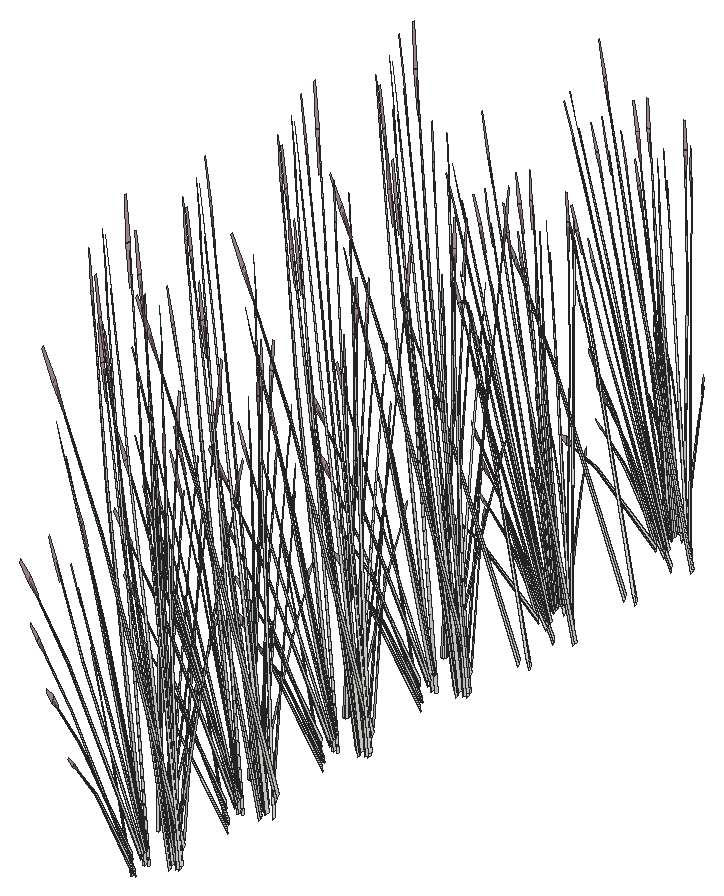
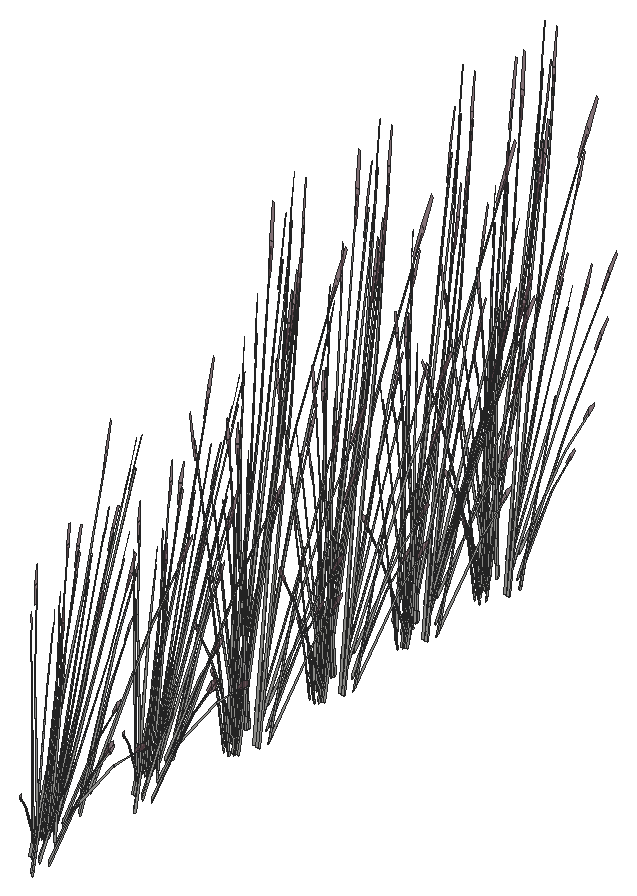
# SketchUp Ruby script. Lengths in inches.
U = 1.inch
M = Sketchup.active_model
def pt(a) = Geom::Point3d.new(a.map { |v| v * U })
def face(e, loops, mat)
  f = e.add_face(loops[0].map { |a| pt(a) })
  loops[1..].each { |l| e.add_face(l.map { |a| pt(a) }).erase! }
  f.material = f.back_material = mat if mat
  f
end
# faces: each face lists its corners as indices into pts; further lists are holes
def faces(e, pts, list, mat = nil) = list.each { |f| face(e, (f[0].is_a?(Array) ? f : [f]).map { |l| l.map { |i| pts[i] } }, mat) }
# xy, xz, yz: faces in a plane at the given z, y or x. An outline is a flat list of corners, or four numbers for a rectangle; further outlines are holes
def ring(l) = l.size == 4 ? [[l[0], l[1]], [l[2], l[1]], [l[2], l[3]], [l[0], l[3]]] : l.each_slice(2).to_a
def flat(e, list, mat, &to3) = list.each { |f| face(e, (f[0].is_a?(Array) ? f : [f]).map { |l| ring(l).map { |u, v| to3.(u, v) } }, mat) }
def xy(e, z, list, mat = nil) = flat(e, list, mat) { |x, y| [x, y, z] }
def xz(e, y, list, mat = nil) = flat(e, list, mat) { |x, z| [x, y, z] }
def yz(e, x, list, mat = nil) = flat(e, list, mat) { |y, z| [x, y, z] }
def lines(e, pts, list) = list.each { |a, b| e.add_line(pt(pts[a]), pt(pts[b])) }
# prism: a flat outline (further loops are holes) pulled along v
def prism(e, loops, v, mat = nil)
  f = face(e, loops, mat); d = Geom::Vector3d.new(v.map { |x| x * U })
  f.pushpull(f.normal.samedirection?(d) ? d.length : -d.length)
end
def box(e, o, s, mat = nil) = prism(e, [[o, [o[0] + s[0], o[1], o[2]], [o[0] + s[0], o[1] + s[1], o[2]], [o[0], o[1] + s[1], o[2]]]], [0, 0, s[2]], mat)
def at(x, y, z, deg = 0) = Geom::Transformation.translation(pt([x, y, z])) * Geom::Transformation.rotation(ORIGIN, Z_AXIS, deg.degrees)
def axes(o, x, y, z) = Geom::Transformation.new([*x, 0, *y, 0, *z, 0, *pt(o).to_a, 1])
def part(name) = M.definitions.add(name)
# library, detail: a bought-in or finely detailed component or shape, given as its bounding box
def library(name, o, s) = part(name).tap { |d| box(d.entities, o, s) }
def detail(e, o, s) = box(e.add_group.entities, o, s)
def put(e, d, t, mat = nil) = e.add_instance(d, t).tap { |i| i.material = mat if mat }
def group(e, t, mat = nil) = e.add_group.tap { |g| g.transformation = t; g.material = mat if mat }.entities
root = M.entities
M.materials.add("LightPink_Translucent").color = [144, 107, 117]
M.materials["LightPink_Translucent"].alpha = 0.75
c1 = part("blade")
p = [[2.15,0.21,22],[0,0.17,0],[0.09,0.45,0],[2.18,0.31,22],[2.29,0.31,22],[0.38,0.45,0],
  [2.48,0.24,33],[2.49,0.24,33],[2.48,0.22,33]]
faces(c1.entities,p,[[0,1,2,3],[4,5,2,3],[6,3,4,7],[8,0,3,6]])
c2 = part("seeds")
p = [[0.3,-0.1,1.38],[-0.01,-0.03,1.59],[-0.01,-0.03,0.03],[0.14,-0.07,-0.07],[0.29,-0.03,3],[0.15,0.01,3.11]]
faces(c2.entities,p,[[0,1,2,3],[1,0,4,5]],"LightPink_Translucent")
c3 = part("blade with seeds")
put(c3.entities,c1,at(0,0,0))
put(c3.entities,c2,axes([2.4,0.25,30.99],[1.5799,-0.05474,1.17369],[-0.12525,1.92788,0.29478],[-0.07173,-0.02425,1.56792]))
put(root,c3,axes([402.11,21.07,-7.6],[0.02575,-0.41332,0.05988],[0.38885,0.01133,0.47138],[-0.14895,-0.04325,0.71878]))
put(root,c3,axes([402.13,36.38,-10.12],[-0.47863,-0.27177,-0.46235],[0.28609,-0.48733,0],[-0.10901,-0.0619,1.46668]))
put(root,c3,axes([401.1875,24.6,-7.61],[-0.01271,0.10756,1.62908],[0.36076,0.37419,-0.25764],[-0.09444,0.17695,0.13065]))
put(root,c3,axes([402.15,48.24,-10.12],[-0.47863,-0.27177,-0.46235],[0.28609,-0.48733,0],[-0.10901,-0.0619,1.46668]))
put(root,c3,axes([401.92,32.34,-10.61],[-0.04954,0.0716,1.6421],[-0.50062,0.15438,-0.25086],[-0.12094,-0.14044,0.2797]))
put(root,c3,axes([401.36,35.34,-7.3125],[0.47307,0.29971,-0.11324],[-0.27254,0.43404,-0.62851],[-0.13365,0.15087,0.95501]))
put(root,c3,axes([401.94,44.19,-10.61],[-0.04954,0.0716,1.6421],[-0.50062,0.15438,-0.25086],[-0.12094,-0.14044,0.2797]))
put(root,c3,axes([401.38,47.2,-7.3125],[0.47307,0.29971,-0.11324],[-0.27254,0.43404,-0.62851],[-0.13365,0.15087,0.95501]))
put(root,c3,axes([403.21,23.36,-10.08],[-0.53199,-0.08911,-0.58063],[0.11226,-0.54969,-0.15239],[-0.15876,-0.06661,1.28164]))
put(root,c3,axes([403.3,20.36,-6.94],[-0.34131,0.52108,-0.12682],[-0.49429,-0.3002,-0.70393],[-0.17182,-0.14722,1.06961]))
put(root,c3,axes([400.33,14.06,-6.74],[0.45129,0.14509,-0.06041],[-0.13882,0.44656,-0.27392],[-0.07381,0.0678,0.90349]))
put(root,c3,axes([402.42,36.71,-9.79],[-0.31974,0.54466,0],[-0.53494,-0.30375,-0.48057],[-0.12184,-0.06918,1.52448]))
put(root,c3,axes([402.37,21.38,-7.3],[0.29098,0.34031,0.32977],[-0.33226,0.32215,-0.42575],[-0.16881,-0.04902,0.81462]))
put(root,c3,axes([401.95,73.36,-7.62],[0.06527,0.01458,1.65179],[0.20191,0.48025,-0.15608],[-0.1336,0.12605,0.29231]))
put(root,c3,axes([402.45,48.57,-9.79],[-0.31974,0.54466,0],[-0.53494,-0.30375,-0.48057],[-0.12184,-0.06918,1.52448]))
put(root,c3,axes([401.96,59.11,-7.62],[0.06527,0.01458,1.65179],[0.20191,0.48025,-0.15608],[-0.1336,0.12605,0.29231]))
put(root,c3,axes([403.4375,72.77,-7.64],[-0.13855,0.49442,-0.47583],[-0.47502,-0.16947,-0.36857],[-0.19125,0.04534,0.91046]))
put(root,c3,axes([403.44,58.52,-7.64],[-0.13855,0.49442,-0.47583],[-0.47502,-0.16947,-0.36857],[-0.19125,0.04534,0.91046]))
put(root,c3,axes([401.34,12.8,-7.3],[0.44516,-0.07768,0.32977],[0.11755,0.44407,-0.42575],[-0.12757,0.11927,0.81462]))
put(root,c3,axes([403.15,20.78,-7.36],[-0.43608,-0.26272,-0.66157],[0.30991,-0.46038,0.07984],[-0.158,-0.15687,0.93586]))
put(root,c3,axes([402.95,20.79,-7.64],[-0.50465,0.12921,-0.47583],[-0.08828,-0.48932,-0.36857],[-0.13555,-0.14022,0.91046]))
put(root,c3,axes([401.6,14.92,-9.59],[0.16138,-0.08575,1.33163],[0.39845,0.25854,-0.28638],[-0.1186,0.22371,0.56934]))
put(root,c3,axes([403.8,71.7,-7.64],[-0.37135,0.36005,-0.47583],[-0.32522,-0.38035,-0.36857],[-0.18868,-0.05478,0.91046]))
put(root,c3,axes([403.8,57.46,-7.64],[-0.37135,0.36005,-0.47583],[-0.32522,-0.38035,-0.36857],[-0.18868,-0.05478,0.91046]))
put(root,c3,axes([403.2,72.74,-10.61],[0.01297,0.08566,1.6421],[-0.26146,0.44735,-0.25086],[-0.18572,-0.02255,0.2797]))
put(root,c3,axes([403.21,58.49,-10.61],[0.01297,0.08566,1.6421],[-0.26146,0.44735,-0.25086],[-0.18572,-0.02255,0.2797]))
put(root,c3,axes([401.37,10.03,-10.02],[-0.14753,0.44383,-0.03625],[-0.45406,-0.13653,-0.16435],[-0.06894,-0.07259,0.54209]))
put(root,c3,axes([400.58,36.65,-6.74],[0.45129,0.14509,-0.06041],[-0.13882,0.44656,-0.27392],[-0.07381,0.0678,0.90349]))
put(root,c3,axes([400.6,48.5,-6.74],[0.45129,0.14509,-0.06041],[-0.13882,0.44656,-0.27392],[-0.07381,0.0678,0.90349]))
put(root,c3,axes([402.51,24.4,-10.12],[-0.47863,-0.27177,-0.46235],[0.28609,-0.48733,0],[-0.10901,-0.0619,1.46668]))
put(root,c3,axes([402.55,8.52,-7.62],[-0.00954,0.06515,1.65179],[-0.47055,0.23645,-0.15608],[-0.13847,-0.12087,0.29231]))
put(root,c3,axes([402.3,20.35,-10.61],[-0.04954,0.0716,1.6421],[-0.50062,0.15438,-0.25086],[-0.12094,-0.14044,0.2797]))
put(root,c3,axes([401.73,23.36,-7.3125],[0.47307,0.29971,-0.11324],[-0.27254,0.43404,-0.62851],[-0.13365,0.15087,0.95501]))
put(root,c3,axes([403.27,70.69,-7.62],[0.03791,0.05424,1.65179],[-0.18278,0.48761,-0.15608],[-0.18511,0.00353,0.29231]))
put(root,c3,axes([401.59,35.38,-7.3],[0.44516,-0.07768,0.32977],[0.11755,0.44407,-0.42575],[-0.12757,0.11927,0.81462]))
put(root,c3,axes([403.28,56.45,-7.62],[0.03791,0.05424,1.65179],[-0.18278,0.48761,-0.15608],[-0.18511,0.00353,0.29231]))
put(root,c3,axes([401.61,47.24,-7.3],[0.44516,-0.07768,0.32977],[0.11755,0.44407,-0.42575],[-0.12757,0.11927,0.81462]))
put(root,c3,axes([402.05,9.47,-9.59],[-0.03097,0.17781,1.33163],[-0.45273,0.14885,-0.28638],[-0.10583,-0.22982,0.56934]))
put(root,c3,axes([401.84,37.5,-9.59],[0.16138,-0.08575,1.33163],[0.39845,0.25854,-0.28638],[-0.1186,0.22371,0.56934]))
put(root,c3,axes([402.8,24.72,-9.79],[-0.31974,0.54466,0],[-0.53494,-0.30375,-0.48057],[-0.12184,-0.06918,1.52448]))
put(root,c3,axes([401.86,49.36,-9.59],[0.16138,-0.08575,1.33163],[0.39845,0.25854,-0.28638],[-0.1186,0.22371,0.56934]))
put(root,c3,axes([402.5,74.88,-9.42],[0.21313,-0.24635,1.06958],[0.0841,0.38999,0.78586],[-0.15402,0.06983,0.23558]))
put(root,c3,axes([402.19,9.93,-8.39],[0.1169,0.17452,1.59586],[-0.54019,0.14692,0.12904],[-0.12209,-0.27397,0.68222]))
put(root,c3,axes([402.51,60.64,-9.42],[0.21313,-0.24635,1.06958],[0.0841,0.38999,0.78586],[-0.15402,0.06983,0.23558]))
put(root,c3,axes([401.61,32.61,-10.02],[-0.14753,0.44383,-0.03625],[-0.45406,-0.13653,-0.16435],[-0.06894,-0.07259,0.54209]))
put(root,c3,axes([403.19,12.84,-9.52],[-0.51635,0.36087,-0.27094],[-0.34336,-0.5099,-0.46562],[-0.1274,-0.05178,1.4872]))
put(root,c3,axes([401.63,44.47,-10.02],[-0.14753,0.44383,-0.03625],[-0.45406,-0.13653,-0.16435],[-0.06894,-0.07259,0.54209]))
put(root,c3,axes([403.7,70.37,-7.61],[-0.11004,-0.00384,1.62908],[-0.35032,0.38367,-0.25764],[-0.18692,-0.07839,0.13065]))
put(root,c3,axes([403.7,56.12,-7.61],[-0.11004,-0.00384,1.62908],[-0.35032,0.38367,-0.25764],[-0.18692,-0.07839,0.13065]))
put(root,c3,axes([401.76,13.98,-7.59],[-0.36417,-0.37086,0.447],[0.38674,-0.31985,0.36857],[-0.06718,0.174,0.92496]))
put(root,c3,axes([402.38,9.84,-7.78],[-0.07899,-0.43781,-0.32977],[0.45153,-0.11561,0.42575],[-0.12128,-0.12546,0.81462]))
put(root,c3,axes([403.25,72.49,-7.59],[0.14449,-0.4956,0.447],[0.47502,0.16947,0.36857],[-0.1868,0.02978,0.92496]))
put(root,c3,axes([402.79,31.11,-7.62],[-0.00954,0.06515,1.65179],[-0.47055,0.23645,-0.15608],[-0.13847,-0.12087,0.29231]))
put(root,c3,axes([403.25,58.24,-7.59],[0.14449,-0.4956,0.447],[0.47502,0.16947,0.36857],[-0.1868,0.02978,0.92496]))
put(root,c3,axes([402.82,42.96,-7.62],[-0.00954,0.06515,1.65179],[-0.47055,0.23645,-0.15608],[-0.13847,-0.12087,0.29231]))
put(root,c3,axes([401.125,12.05,-9.79],[-0.63949,0,0],[0,-0.60749,-0.48057],[0,-0.13836,1.52448]))
put(root,c3,axes([402.02,13.6,-10.11],[-0.12013,-0.47362,-0.28847],[0.47712,-0.13449,0.28847],[-0.09619,-0.05462,1.29413]))
put(root,c3,axes([403.42,72.35,-7.3125],[0.25732,0.49218,-0.11324],[-0.45669,0.24187,-0.62851],[-0.19245,0.06494,0.95501]))
put(root,c3,axes([403.42,58.1,-7.3125],[0.25732,0.49218,-0.11324],[-0.45669,0.24187,-0.62851],[-0.19245,0.06494,0.95501]))
put(root,c3,axes([401.63,13.94,-7.6],[-0.42027,-0.02533,0.05988],[0.01152,-0.38243,0.47138],[-0.04398,0.14649,0.71878]))
put(root,c3,axes([403.99,71.32,-7.3125],[-0.02738,0.55277,-0.11324],[-0.51847,-0.01511,-0.62851],[-0.19968,-0.0384,0.95501]))
put(root,c3,axes([402.29,32.05,-9.59],[-0.03097,0.17781,1.33163],[-0.45273,0.14885,-0.28638],[-0.10583,-0.22982,0.56934]))
put(root,c3,axes([400.95,24.66,-6.74],[0.45129,0.14509,-0.06041],[-0.13882,0.44656,-0.27392],[-0.07381,0.0678,0.90349]))
put(root,c3,axes([404,57.08,-7.3125],[-0.02738,0.55277,-0.11324],[-0.51847,-0.01511,-0.62851],[-0.19968,-0.0384,0.95501]))
put(root,c3,axes([403.66,71.36,-7.78],[-0.29098,-0.34031,-0.32977],[0.33226,-0.32215,0.42575],[-0.16881,-0.04902,0.81462]))
put(root,c3,axes([402.3125,43.91,-9.59],[-0.03097,0.17781,1.33163],[-0.45273,0.14885,-0.28638],[-0.10583,-0.22982,0.56934]))
put(root,c3,axes([403.67,57.12,-7.78],[-0.29098,-0.34031,-0.32977],[0.33226,-0.32215,0.42575],[-0.16881,-0.04902,0.81462]))
put(root,c3,axes([403.21,72.36,-7.6],[-0.18783,-0.37061,0.05988],[0.34252,-0.1814,0.47138],[-0.15099,0.03579,0.71878]))
put(root,c3,axes([403.22,58.11,-7.6],[-0.18783,-0.37061,0.05988],[0.34252,-0.1814,0.47138],[-0.15099,0.03579,0.71878]))
put(root,c3,axes([402.4375,32.51,-8.39],[0.1169,0.17452,1.59586],[-0.54019,0.14692,0.12904],[-0.12209,-0.27397,0.68222]))
put(root,c3,axes([401.76,14.09,-7.78],[-0.34603,0.28618,-0.32977],[-0.32756,-0.32677,0.42575],[-0.04984,0.16603,0.81462]))
put(root,c3,axes([402.46,44.37,-8.39],[0.1169,0.17452,1.59586],[-0.54019,0.14692,0.12904],[-0.12209,-0.27397,0.68222]))
put(root,c3,axes([403.43,35.42,-9.52],[-0.51635,0.36087,-0.27094],[-0.34336,-0.5099,-0.46562],[-0.1274,-0.05178,1.4872]))
put(root,c3,axes([404.07,73.38,-8.39],[0.12773,-0.16701,1.59586],[0.32252,0.4508,0.12904],[-0.22121,0.20529,0.68222]))
put(root,c3,axes([401.96,23.4,-7.3],[0.44516,-0.07768,0.32977],[0.11755,0.44407,-0.42575],[-0.12757,0.11927,0.81462]))
put(root,c3,axes([404.08,59.14,-8.39],[0.12773,-0.16701,1.59586],[0.32252,0.4508,0.12904],[-0.22121,0.20529,0.68222]))
put(root,c3,axes([403.3,73.82,-7.78],[-0.44516,0.07768,-0.32977],[-0.11755,-0.44407,0.42575],[-0.12757,0.11927,0.81462]))
put(root,c3,axes([403.31,59.57,-7.78],[-0.44516,0.07768,-0.32977],[-0.11755,-0.44407,0.42575],[-0.12757,0.11927,0.81462]))
put(root,c3,axes([403.46,47.28,-9.52],[-0.51635,0.36087,-0.27094],[-0.34336,-0.5099,-0.46562],[-0.1274,-0.05178,1.4872]))
put(root,c3,axes([402.01,36.5625,-7.59],[-0.36417,-0.37086,0.447],[0.38674,-0.31985,0.36857],[-0.06718,0.174,0.92496]))
put(root,c3,axes([402.03,48.42,-7.59],[-0.36417,-0.37086,0.447],[0.38674,-0.31985,0.36857],[-0.06718,0.174,0.92496]))
put(root,c3,axes([402.22,25.51,-9.59],[0.16138,-0.08575,1.33163],[0.39845,0.25854,-0.28638],[-0.1186,0.22371,0.56934]))
put(root,c3,axes([402.625,32.42,-7.78],[-0.07899,-0.43781,-0.32977],[0.45153,-0.11561,0.42575],[-0.12128,-0.12546,0.81462]))
put(root,c3,axes([403.06,75.14,-10.61],[0.0686,0.0543,1.6421],[0.11632,0.50315,-0.25086],[-0.15204,0.10729,0.2797]))
put(root,c3,axes([401.99,20.625,-10.02],[-0.14753,0.44383,-0.03625],[-0.45406,-0.13653,-0.16435],[-0.06894,-0.07259,0.54209]))
put(root,c3,axes([402.65,44.28,-7.78],[-0.07899,-0.43781,-0.32977],[0.45153,-0.11561,0.42575],[-0.12128,-0.12546,0.81462]))
put(root,c3,axes([403.07,60.89,-10.61],[0.0686,0.0543,1.6421],[0.11632,0.50315,-0.25086],[-0.15204,0.10729,0.2797]))
put(root,c3,axes([401.37,34.64,-9.79],[-0.63949,0,0],[0,-0.60749,-0.48057],[0,-0.13836,1.52448]))
put(root,c3,axes([403.53,13.23,-10.08],[-0.34446,0.40855,-0.58063],[-0.42791,-0.37046,-0.15239],[-0.13803,0.10191,1.28164]))
put(root,c3,axes([402.27,36.18,-10.11],[-0.12013,-0.47362,-0.28847],[0.47712,-0.13449,0.28847],[-0.09619,-0.05462,1.29413]))
put(root,c3,axes([401.39,46.5,-9.79],[-0.63949,0,0],[0,-0.60749,-0.48057],[0,-0.13836,1.52448]))
put(root,c3,axes([402.96,72.18,-9.42],[0.3265,-0.03889,1.06958],[-0.20711,0.3427,0.78586],[-0.16135,-0.05141,0.23558]))
put(root,c3,axes([402.29,48.04,-10.11],[-0.12013,-0.47362,-0.28847],[0.47712,-0.13449,0.28847],[-0.09619,-0.05462,1.29413]))
put(root,c3,axes([401.875,36.53,-7.6],[-0.42027,-0.02533,0.05988],[0.01152,-0.38243,0.47138],[-0.04398,0.14649,0.71878]))
put(root,c3,axes([402.65,10.19,-7.3],[0.07899,0.43781,0.32977],[-0.45153,0.11561,-0.42575],[-0.12128,-0.12546,0.81462]))
put(root,c3,axes([402.97,57.93,-9.42],[0.3265,-0.03889,1.06958],[-0.20711,0.3427,0.78586],[-0.16135,-0.05141,0.23558]))
put(root,c3,axes([401.9,48.39,-7.6],[-0.42027,-0.02533,0.05988],[0.01152,-0.38243,0.47138],[-0.04398,0.14649,0.71878]))
put(root,c3,axes([400.53,15.11,-7.62],[0.05802,-0.03282,1.65179],[0.47954,0.21828,-0.15608],[-0.01127,0.18175,0.29231]))
put(root,c3,axes([401.62,11.89,-9.83],[-0.47569,0.45698,0.2864],[-0.47598,-0.45217,-0.33981],[-0.01661,-0.12977,1.53541]))
put(root,c3,axes([402.01,36.67,-7.78],[-0.34603,0.28618,-0.32977],[-0.32756,-0.32677,0.42575],[-0.04984,0.16603,0.81462]))
put(root,c3,axes([403.17,19.12,-7.62],[-0.00954,0.06515,1.65179],[-0.47055,0.23645,-0.15608],[-0.13847,-0.12087,0.29231]))
put(root,c3,axes([402.03,48.53,-7.78],[-0.34603,0.28618,-0.32977],[-0.32756,-0.32677,0.42575],[-0.04984,0.16603,0.81462]))
put(root,c3,axes([405.76,50.98,-8.39],[0.21212,-0.01231,1.59586],[-0.14072,0.53355,0.12904],[-0.3023,-0.033,0.68222]))
put(root,c3,axes([405.77,63.82,-8.39],[0.21212,-0.01231,1.59586],[-0.14072,0.53355,0.12904],[-0.3023,-0.033,0.68222]))
put(root,c3,axes([402.66,20.06,-9.59],[-0.03097,0.17781,1.33163],[-0.45273,0.14885,-0.28638],[-0.10583,-0.22982,0.56934]))
put(root,c3,axes([403.58,13.15,-8.9],[0.44194,0.21918,1.40854],[-0.43295,0.47219,0.557],[-0.19393,-0.27986,1.18082]))
put(root,c3,axes([403.36,73.72,-7.59],[-0.12683,-0.50025,0.447],[0.49754,-0.08682,0.36857],[-0.14663,0.11765,0.92496]))
put(root,c3,axes([403.37,59.48,-7.59],[-0.12683,-0.50025,0.447],[0.49754,-0.08682,0.36857],[-0.14663,0.11765,0.92496]))
put(root,c3,axes([402.8125,20.53,-8.39],[0.1169,0.17452,1.59586],[-0.54019,0.14692,0.12904],[-0.12209,-0.27397,0.68222]))
put(root,c3,axes([403.81,23.4375,-9.52],[-0.51635,0.36087,-0.27094],[-0.34336,-0.5099,-0.46562],[-0.1274,-0.05178,1.4872]))
put(root,c3,axes([401.89,9.18,-9.42],[0.26677,0.18918,1.06958],[-0.38851,0.11372,0.78586],[-0.08313,-0.14539,0.23558]))
put(root,c3,axes([403.78,35.82,-10.08],[-0.34446,0.40855,-0.58063],[-0.42791,-0.37046,-0.15239],[-0.13803,0.10191,1.28164]))
put(root,c3,axes([403.77,13,-9.7],[-0.49938,-0.43748,-0.23459],[0.42021,-0.49126,0.51337],[-0.13447,0.05118,1.56642]))
put(root,c3,axes([403.62,71.23,-7.26],[0.42234,-0.40113,0.50064],[0.36424,0.42599,0.4128],[-0.19815,-0.07399,1.03595]))
put(root,c3,axes([403.8,47.68,-10.08],[-0.34446,0.40855,-0.58063],[-0.42791,-0.37046,-0.15239],[-0.13803,0.10191,1.28164]))
put(root,c3,axes([402.86,12.58,-9.94],[-0.30722,-0.45622,-0.41661],[0.46535,-0.32126,0.2005],[-0.09942,-0.05645,1.33761]))
put(root,c3,axes([402.89,32.78,-7.3],[0.07899,0.43781,0.32977],[-0.45153,0.11561,-0.42575],[-0.12128,-0.12546,0.81462]))
put(root,c3,axes([403.625,56.99,-7.26],[0.42234,-0.40113,0.50064],[0.36424,0.42599,0.4128],[-0.19815,-0.07399,1.03595]))
put(root,c3,axes([402.38,24.58,-7.59],[-0.36417,-0.37086,0.447],[0.38674,-0.31985,0.36857],[-0.06718,0.174,0.92496]))
put(root,c3,axes([402.92,44.64,-7.3],[0.07899,0.43781,0.32977],[-0.45153,0.11561,-0.42575],[-0.12128,-0.12546,0.81462]))
put(root,c3,axes([400.77,37.69,-7.62],[0.05802,-0.03282,1.65179],[0.47954,0.21828,-0.15608],[-0.01127,0.18175,0.29231]))
put(root,c3,axes([403.26,73.625,-7.6],[-0.35109,-0.22859,0.05988],[0.2044,-0.32553,0.47138],[-0.11256,0.10524,0.71878]))
put(root,c3,axes([403.27,59.38,-7.6],[-0.35109,-0.22859,0.05988],[0.2044,-0.32553,0.47138],[-0.11256,0.10524,0.71878]))
put(root,c3,axes([400.79,49.55,-7.62],[0.05802,-0.03282,1.65179],[0.47954,0.21828,-0.15608],[-0.01127,0.18175,0.29231]))
put(root,c3,axes([401.86,34.48,-9.83],[-0.47569,0.45698,0.2864],[-0.47598,-0.45217,-0.33981],[-0.01661,-0.12977,1.53541]))
put(root,c3,axes([403,20.43,-7.78],[-0.07899,-0.43781,-0.32977],[0.45153,-0.11561,0.42575],[-0.12128,-0.12546,0.81462]))
put(root,c3,axes([401.99,13.79,-7.03],[-0.01331,0.50278,-0.73435],[-0.56035,-0.03377,0.08862],[-0.05914,0.213,1.03881]))
put(root,c3,axes([401.89,46.34,-9.83],[-0.47569,0.45698,0.2864],[-0.47598,-0.45217,-0.33981],[-0.01661,-0.12977,1.53541]))
put(root,c3,axes([401.74,22.65,-9.79],[-0.63949,0,0],[0,-0.60749,-0.48057],[0,-0.13836,1.52448]))
put(root,c3,axes([402.64,24.19,-10.11],[-0.12013,-0.47362,-0.28847],[0.47712,-0.13449,0.28847],[-0.09619,-0.05462,1.29413]))
put(root,c3,axes([402.25,24.54,-7.6],[-0.42027,-0.02533,0.05988],[0.01152,-0.38243,0.47138],[-0.04398,0.14649,0.71878]))
put(root,c3,axes([401.98,15.2,-9.42],[-0.01324,-0.32319,1.06958],[0.33072,0.23052,0.78586],[-0.06504,0.15405,0.23558]))
put(root,c3,axes([403.82,35.74,-8.9],[0.44194,0.21918,1.40854],[-0.43295,0.47219,0.557],[-0.19393,-0.27986,1.18082]))
put(root,c3,axes([402.45,9.68,-7.26],[0.56969,-0.13971,0.50064],[0.09887,0.54803,0.4128],[-0.13398,-0.16152,1.03595]))
put(root,c3,axes([403.84,47.6,-8.9],[0.44194,0.21918,1.40854],[-0.43295,0.47219,0.557],[-0.19393,-0.27986,1.18082]))
put(root,c3,axes([403.52,12.91,-9.94],[-0.55535,0.03355,-0.41661],[-0.05022,-0.55698,0.2005],[-0.09942,0.05645,1.33761]))
put(root,c3,axes([402.38,24.6875,-7.78],[-0.34603,0.28618,-0.32977],[-0.32756,-0.32677,0.42575],[-0.04984,0.16603,0.81462]))
put(root,c3,axes([403.98,73.79,-8.39],[0.09522,-0.18683,1.59586],[0.39947,0.38663,0.12904],[-0.18021,0.24097,0.68222]))
put(root,c3,axes([402.13,31.76,-9.42],[0.26677,0.18918,1.06958],[-0.38851,0.11372,0.78586],[-0.08313,-0.14539,0.23558]))
put(root,c3,axes([403.98,59.55,-8.39],[0.09522,-0.18683,1.59586],[0.39947,0.38663,0.12904],[-0.18021,0.24097,0.68222]))
put(root,c3,axes([404.01,35.59,-9.7],[-0.49938,-0.43748,-0.23459],[0.42021,-0.49126,0.51337],[-0.13447,0.05118,1.56642]))
put(root,c3,axes([402.16,43.625,-9.42],[0.26677,0.18918,1.06958],[-0.38851,0.11372,0.78586],[-0.08313,-0.14539,0.23558]))
put(root,c3,axes([403.11,35.17,-9.94],[-0.30722,-0.45622,-0.41661],[0.46535,-0.32126,0.2005],[-0.09942,-0.05645,1.33761]))
put(root,c3,axes([404.04,47.45,-9.7],[-0.49938,-0.43748,-0.23459],[0.42021,-0.49126,0.51337],[-0.13447,0.05118,1.56642]))
put(root,c3,axes([403.13,47.03,-9.94],[-0.30722,-0.45622,-0.41661],[0.46535,-0.32126,0.2005],[-0.09942,-0.05645,1.33761]))
put(root,c3,axes([402.24,36.37,-7.03],[-0.01331,0.50278,-0.73435],[-0.56035,-0.03377,0.08862],[-0.05914,0.213,1.03881]))
put(root,c3,axes([402.58,9.8,-7.6],[0.23243,-0.34529,0.05988],[0.331,0.20103,0.47138],[-0.10701,-0.1107,0.71878]))
put(root,c3,axes([402.26,48.23,-7.03],[-0.01331,0.50278,-0.73435],[-0.56035,-0.03377,0.08862],[-0.05914,0.213,1.03881]))
put(root,c3,axes([404.15,23.83,-10.08],[-0.34446,0.40855,-0.58063],[-0.42791,-0.37046,-0.15239],[-0.13803,0.10191,1.28164]))
put(root,c3,axes([403.6,72.49,-7.3],[0.42502,0.15163,0.32977],[-0.12396,0.44238,-0.42575],[-0.17112,0.04056,0.81462]))
put(root,c3,axes([403.6,58.25,-7.3],[0.42502,0.15163,0.32977],[-0.12396,0.44238,-0.42575],[-0.17112,0.04056,0.81462]))
put(root,c3,axes([403.27,20.79,-7.3],[0.07899,0.43781,0.32977],[-0.45153,0.11561,-0.42575],[-0.12128,-0.12546,0.81462]))
put(root,c3,axes([405.85,51.91,-8.39],[0.17745,-0.11497,1.59586],[0.14939,0.53127,0.12904],[-0.27857,0.12007,0.68222]))
put(root,c3,axes([402.23,37.79,-9.42],[-0.01324,-0.32319,1.06958],[0.33072,0.23052,0.78586],[-0.06504,0.15405,0.23558]))
put(root,c3,axes([405.86,64.76,-8.39],[0.17745,-0.11497,1.59586],[0.14939,0.53127,0.12904],[-0.27857,0.12007,0.68222]))
put(root,c3,axes([402.69,32.26,-7.26],[0.56969,-0.13971,0.50064],[0.09887,0.54803,0.4128],[-0.13398,-0.16152,1.03595]))
put(root,c3,axes([402.46,13.84,-9.69],[0.47863,0.27177,0.46235],[-0.28609,0.48733,0],[-0.10901,-0.0619,1.46668]))
put(root,c3,axes([402.25,49.65,-9.42],[-0.01324,-0.32319,1.06958],[0.33072,0.23052,0.78586],[-0.06504,0.15405,0.23558]))
put(root,c3,axes([401.15,25.71,-7.62],[0.05802,-0.03282,1.65179],[0.47954,0.21828,-0.15608],[-0.01127,0.18175,0.29231]))
put(root,c3,axes([402.71,44.12,-7.26],[0.56969,-0.13971,0.50064],[0.09887,0.54803,0.4128],[-0.13398,-0.16152,1.03595]))
put(root,c3,axes([401.81,14.5,-8.87],[0.01124,-0.2806,1.43727],[0.50537,0.14821,0.19862],[-0.04379,0.29905,0.67868]))
put(root,c3,axes([403.76,35.5,-9.94],[-0.55535,0.03355,-0.41661],[-0.05022,-0.55698,0.2005],[-0.09942,0.05645,1.33761]))
put(root,c3,axes([402.24,22.49,-9.83],[-0.47569,0.45698,0.2864],[-0.47598,-0.45217,-0.33981],[-0.01661,-0.12977,1.53541]))
put(root,c3,axes([403.78,47.35,-9.94],[-0.55535,0.03355,-0.41661],[-0.05022,-0.55698,0.2005],[-0.09942,0.05645,1.33761]))
put(root,c3,axes([403.67,73.87,-7.64],[0.13138,0.49631,-0.47583],[-0.49754,0.08682,-0.36857],[-0.14258,0.13331,0.91046]))
put(root,c3,axes([403.68,59.625,-7.64],[0.13138,0.49631,-0.47583],[-0.49754,0.08682,-0.36857],[-0.14258,0.13331,0.91046]))
put(root,c3,axes([402.91,12.84,-9.73],[0.13555,-0.64407,-0.21817],[0.64269,0.11227,0.47743],[-0.1123,-0.08895,1.45677]))
put(root,c3,axes([405.3,52.82,-9.59],[0.17773,0.04462,1.33163],[0.11455,0.45576,-0.28638],[-0.24142,0.08531,0.56934]))
put(root,c3,axes([405.31,65.66,-9.59],[0.17773,0.04462,1.33163],[0.11455,0.45576,-0.28638],[-0.24142,0.08531,0.56934]))
put(root,c3,axes([403.81,71.23,-7.6],[0.02575,-0.41332,0.05988],[0.38885,0.01133,0.47138],[-0.14895,-0.04325,0.71878]))
put(root,c3,axes([404.2,23.75,-8.9],[0.44194,0.21918,1.40854],[-0.43295,0.47219,0.557],[-0.19393,-0.27986,1.18082]))
put(root,c3,axes([403.82,56.99,-7.6],[0.02575,-0.41332,0.05988],[0.38885,0.01133,0.47138],[-0.14895,-0.04325,0.71878]))
put(root,c3,axes([402.89,74.76,-7.61],[-0.01271,0.10756,1.62908],[0.36076,0.37419,-0.25764],[-0.09444,0.17695,0.13065]))
put(root,c3,axes([402.9,60.52,-7.61],[-0.01271,0.10756,1.62908],[0.36076,0.37419,-0.25764],[-0.09444,0.17695,0.13065]))
put(root,c3,axes([402.82,32.38,-7.6],[0.23243,-0.34529,0.05988],[0.331,0.20103,0.47138],[-0.10701,-0.1107,0.71878]))
put(root,c3,axes([404.91,73.51,-10.08],[-0.53199,-0.08911,-0.58063],[0.11226,-0.54969,-0.15239],[-0.15876,-0.06661,1.28164]))
put(root,c3,axes([404.92,59.27,-10.08],[-0.53199,-0.08911,-0.58063],[0.11226,-0.54969,-0.15239],[-0.15876,-0.06661,1.28164]))
put(root,c3,axes([405.01,70.52,-6.94],[-0.34131,0.52108,-0.12682],[-0.49429,-0.3002,-0.70393],[-0.17182,-0.14722,1.06961]))
put(root,c3,axes([405.01,56.27,-6.94],[-0.34131,0.52108,-0.12682],[-0.49429,-0.3002,-0.70393],[-0.17182,-0.14722,1.06961]))
